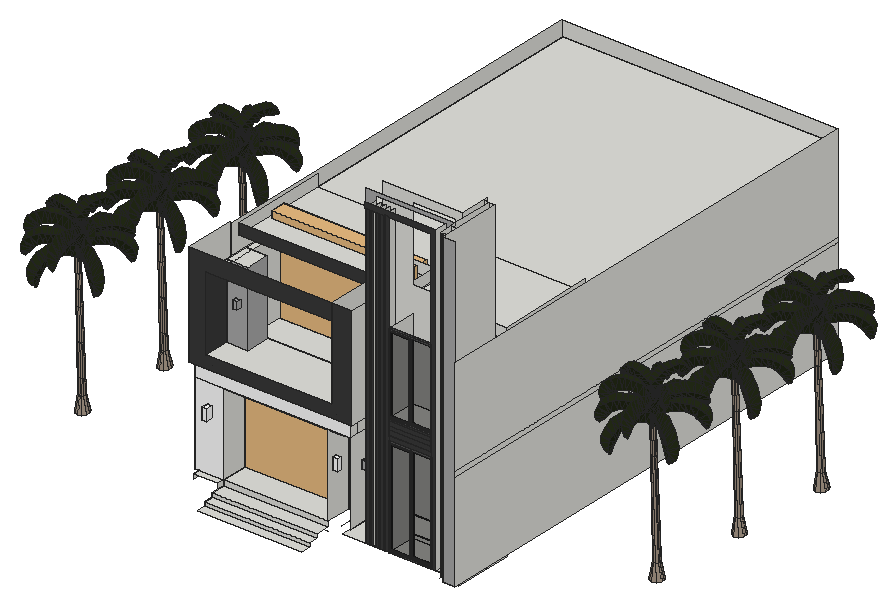
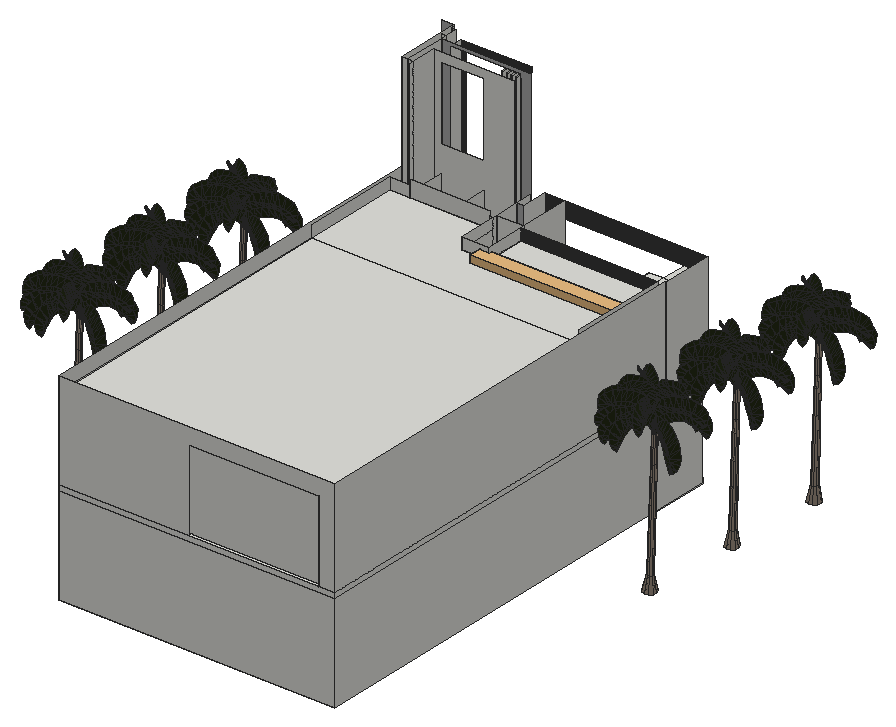
# SketchUp Ruby script. Lengths in inches.
U = 1.inch
M = Sketchup.active_model
def pt(a) = Geom::Point3d.new(a.map { |v| v * U })
def face(e, loops, mat)
  f = e.add_face(loops[0].map { |a| pt(a) })
  loops[1..].each { |l| e.add_face(l.map { |a| pt(a) }).erase! }
  f.material = f.back_material = mat if mat
  f
end
# faces: each face lists its corners as indices into pts; further lists are holes
def faces(e, pts, list, mat = nil) = list.each { |f| face(e, (f[0].is_a?(Array) ? f : [f]).map { |l| l.map { |i| pts[i] } }, mat) }
# xy, xz, yz: faces in a plane at the given z, y or x. An outline is a flat list of corners, or four numbers for a rectangle; further outlines are holes
def ring(l) = l.size == 4 ? [[l[0], l[1]], [l[2], l[1]], [l[2], l[3]], [l[0], l[3]]] : l.each_slice(2).to_a
def flat(e, list, mat, &to3) = list.each { |f| face(e, (f[0].is_a?(Array) ? f : [f]).map { |l| ring(l).map { |u, v| to3.(u, v) } }, mat) }
def xy(e, z, list, mat = nil) = flat(e, list, mat) { |x, y| [x, y, z] }
def xz(e, y, list, mat = nil) = flat(e, list, mat) { |x, z| [x, y, z] }
def yz(e, x, list, mat = nil) = flat(e, list, mat) { |y, z| [x, y, z] }
def lines(e, pts, list) = list.each { |a, b| e.add_line(pt(pts[a]), pt(pts[b])) }
# prism: a flat outline (further loops are holes) pulled along v
def prism(e, loops, v, mat = nil)
  f = face(e, loops, mat); d = Geom::Vector3d.new(v.map { |x| x * U })
  f.pushpull(f.normal.samedirection?(d) ? d.length : -d.length)
end
def box(e, o, s, mat = nil) = prism(e, [[o, [o[0] + s[0], o[1], o[2]], [o[0] + s[0], o[1] + s[1], o[2]], [o[0], o[1] + s[1], o[2]]]], [0, 0, s[2]], mat)
def at(x, y, z, deg = 0) = Geom::Transformation.translation(pt([x, y, z])) * Geom::Transformation.rotation(ORIGIN, Z_AXIS, deg.degrees)
def axes(o, x, y, z) = Geom::Transformation.new([*x, 0, *y, 0, *z, 0, *pt(o).to_a, 1])
def part(name) = M.definitions.add(name)
# library, detail: a bought-in or finely detailed component or shape, given as its bounding box
def library(name, o, s) = part(name).tap { |d| box(d.entities, o, s) }
def detail(e, o, s) = box(e.add_group.entities, o, s)
def put(e, d, t, mat = nil) = e.add_instance(d, t).tap { |i| i.material = mat if mat }
def group(e, t, mat = nil) = e.add_group.tap { |g| g.transformation = t; g.material = mat if mat }.entities
root = M.entities
M.materials.add("Glass_Tinted_Gray").color = [0, 0, 0]
M.materials["Glass_Tinted_Gray"].alpha = 0.125
M.materials.add("Manila2").color = [36, 43, 22]
M.materials.add("ManilaTruck").color = [158, 143, 128]
M.materials.add("[0135_DarkGray]").color = [81, 81, 81]
M.materials.add("[Color M00]").color = [255, 255, 255]
M.materials.add("[Color M03]").color = [170, 170, 170]
M.materials.add("[Color M06]").color = [86, 86, 86]
M.materials.add("[Color M07]").color = [58, 58, 58]
M.materials.add("[Mirror 02]").color = [229, 229, 229]
M.materials.add("[Terrazzo Light Blue]").color = [196, 214, 227]
c1 = part("P_trunck")
xz(c1.entities,2.71,[[7.39,73.15,8.49,73.15,9.26,91.63,8.16,91.63]],"ManilaTruck")
xz(c1.entities,6.09,[[3.91,10.2,7.39,73.15,8.49,73.15,5.33,10.2],[7.39,73.15,8.16,91.63,9.26,91.63,8.49,73.15]],"ManilaTruck")
p = [[3.19,0,0],[3.91,1.7,10.2],[2.75,2.54,10.2],[0.88,1.68,0],[6.05,0,0],[5.33,1.7,10.2],
  [8.36,1.68,0],[6.49,2.54,10.2],[2.31,3.9,10.2],[0,4.39,0],[9.24,4.39,0],[6.93,3.9,10.2],
  [2.75,5.25,10.2],[0.88,7.11,0],[8.36,7.11,0],[6.49,5.25,10.2],[3.91,6.09,10.2],[3.19,8.79,0],
  [6.05,8.79,0],[5.33,6.09,10.2],[7.39,2.71,73.15],[6.5,3.36,73.15],[8.49,2.71,73.15],[9.38,3.36,73.15],
  [6.16,4.4,73.15],[9.72,4.4,73.15],[6.5,5.45,73.15],[9.38,5.45,73.15],[7.39,6.09,73.15],[8.49,6.09,73.15],
  [8.16,2.71,91.63],[7.27,3.36,91.63],[10.15,3.36,91.63],[9.26,2.71,91.63],[6.93,4.4,91.63],[10.49,4.4,91.63],
  [7.27,5.45,91.63],[10.15,5.45,91.63],[8.16,6.09,91.63],[9.26,6.09,91.63]]
faces(c1.entities,p,[[0,1,2,3],[4,5,1,0],[6,7,5,4],[3,2,8,9],[6,10,11,7],[8,12,13,9],[11,10,14,15],[13,12,16,17],
  [18,19,15,14],[17,16,19,18],[1,20,21,2],[5,22,20,1],[7,23,22,5],[2,21,24,8],[7,11,25,23],[8,24,26,12],
  [11,15,27,25],[12,26,28,16],[19,29,27,15],[20,30,31,21],[23,32,33,22],[31,34,24,21],[23,25,35,32],[34,36,26,24],
  [25,27,37,35],[26,36,38,28],[29,39,37,27]],"ManilaTruck")
c2 = part("halfleave")
p = [[3.15,0,0],[0.57,2.5,1.86],[4.875,1.71,0],[46.16,1.62,0],[42.0625,6.98,0],[45.79,16.25,3.85],
  [48.16,12.12,1.98],[48.16,1.62,0],[6.6,3.42,0],[-0.25,5.68,3.48],[9.02,6.6,0],[-0.31,11.68,4.96],
  [2.05,16.625,5.9],[10.99,8.52,0],[36.71,10.67,0],[41.5,21.18,5.01],[8.2,21.17,6.52],[12.96,10.44,0],
  [15.16,24.88,6.8125],[17.61,12.89,0],[31.19,13.02,0],[36.16,23.66,5.26],[19.91,24.88,6.5625],[20.53,13.55,0],
  [25.77,13.9375,0],[30.57,24.88,6.0625],[25.21,24.88,6.26]]
faces(c2.entities,p,[[0,1,2],[3,4,5],[5,6,3],[7,3,6],[2,1,8],[9,8,1],[8,9,10],[11,10,9],
  [11,12,10],[13,10,12],[4,14,15],[15,5,4],[12,16,13],[17,13,16],[16,18,17],[19,17,18],
  [14,20,21],[21,15,14],[18,22,19],[23,19,22],[20,24,25],[25,21,20],[22,26,23],[24,23,26],
  [26,25,24]],"Manila2")
c3 = part("palmfronmanila")
put(c3.entities,c2,axes([0,0,4.06],[1,0,0],[0,1,0],[0,0,-1]))
put(c3.entities,c2,at(0,0,4.06))
c4 = part("manilafronnew")
put(c4.entities,c3,axes([0,16.76,11.56],[1,0,0],[0,0,1],[0,-1,0]))
c5 = part("Palm tree")
put(c5.entities,c1,axes([-10.55,-3.84,0],[1.24992,0,0],[0,1.28016,0],[0,0,1.424]))
g1 = group(c5.entities,at(-43.54,-39.32,114.59))
put(g1,c4,axes([4.6,65.71,26.23],[0.53953,-0.65683,-0.22776],[0.61942,0.58508,-0.22],[0.31564,-0.02543,0.82105]))
put(g1,c4,axes([82.14,44.18,-7.44],[-0.84198,0.16366,0.22983],[-0.16944,-0.87168,0],[0.22561,-0.04385,0.85774]))
put(g1,c4,axes([74.79,11.41,2.76],[-0.448,0.77596,0],[-0.77596,-0.448,0],[0,0,0.896]))
put(g1,c4,axes([70.64,6.04,20.22],[-0.30809,0.82895,-0.08038],[-0.79676,-0.31832,-0.22889],[-0.24248,-0.00729,0.85422]))
put(g1,c4,axes([56.04,79.09,38.5],[-0.31814,-0.55104,-0.36736],[0.63629,-0.36736,0],[-0.18368,-0.31814,0.63629]))
put(g1,c4,axes([8.39,50.1,50.01],[0.44591,-0.25744,-0.51489],[0.36408,0.63061,0],[0.44591,-0.25744,0.51489]))
put(g1,c4,axes([8.53,12.03,22.52],[0.79394,0.3635,-0.23397],[-0.37632,0.82195,0],[0.21274,0.0974,0.8732]))
put(g1,c4,axes([54.07,81.55,-7.16],[-0.44094,-0.76373,0.19874],[0.78289,-0.452,0],[0.09937,0.17211,0.88188]))
put(g1,c4,axes([11.98,71.79,5.35],[0.444,-0.76903,0],[0.76903,0.444,0],[0,0,0.888]))
put(g1,c4,axes([-0.47,46.08,5.17],[0.83758,-0.34011,0],[0.34011,0.83758,0],[0,0,0.904]))
put(g1,c4,axes([35.85,3.71,-10.8],[0.42686,0.73934,0.2973],[-0.78289,0.452,0],[-0.14865,-0.25747,0.85372]))
put(g1,c4,axes([0.28,29.91,5.17],[0.904,0,0],[0,0.904,0],[0,0,0.904]))
put(g1,c4,axes([82.45,61.59,11.57],[-0.88287,-0.17622,-0.08182],[0.17259,-0.88617,0.04625],[-0.08923,0.02954,0.8991]))
put(g1,c4,axes([59.47,9.58,46.3125],[-0.10851,0.51281,-0.52416],[-0.72522,-0.15346,0],[-0.10851,0.51281,0.52416]))
c6 = part("עצי+דקל")
put(c6.entities,c5,axes([111.95,22.91,0],[1.33,0,0],[0,1.33,0],[0,0,1.33]))
put(c6.entities,c5,axes([230.0625,22.91,0],[1.33,0,0],[0,1.33,0],[0,0,1.33]))
put(c6.entities,c5,axes([348.17,22.91,0],[1.33,0,0],[0,1.33,0],[0,0,1.33]))
c7 = part("PENTEK_RP Fineline 50S_Sliding_DoorCase_E1")
box(c7.entities,[0,0,0],[1.51,3.66,99.27],"[0135_DarkGray]")
c8 = part("PENTEK_RP Fineline 50S_SlidingDooe_Case_E2")
box(c8.entities,[0,0,0],[96.25,3.66,1.51],"[0135_DarkGray]")
c9 = part("pentek_RP Fineline 50S_SlidingDoor_Case")
put(c9.entities,c7,at(97.76,0,0))
put(c9.entities,c8,at(1.51,0,0))
put(c9.entities,c7,at(0,0,0))
put(c9.entities,c8,at(1.51,0,97.76))
c10 = part("PENTEK_RP Fineline 50S_SlidingDoor_GlazingBead_2")
box(c10.entities,[0,0,0],[0.56,0.59,94.39],"[0135_DarkGray]")
c11 = part("PENTEK_RP Fineline 50S_SlidingDoor_Glass")
box(c11.entities,[0,0,0],[46.58,0.16,94.39],"Glass_Tinted_Gray")
c12 = part("PENTEK_RP Fineline 50S_SlidingDoor_GlazingBead")
box(c12.entities,[0,0,0],[45.47,0.59,0.56],"[0135_DarkGray]")
c13 = part("PENTEK_RP Fineline 50S_SlidingDoor_Leaf_E1")
xy(c13.entities,0,[[0,0,0.93,1.97],[0.93,1.57,1.49,1.97]],"[0135_DarkGray]")
xy(c13.entities,96.25,[[0,0,0.93,0,0.93,1.57,1.49,1.57,1.49,1.97,0,1.97]],"[0135_DarkGray]")
xz(c13.entities,0,[[0,0,0.93,96.25]],"[0135_DarkGray]")
xz(c13.entities,1.57,[[0.93,0,1.49,95.32],[0.93,95.32,1.49,96.25]],"[0135_DarkGray]")
xz(c13.entities,1.97,[[0,0,1.49,96.25]],"[0135_DarkGray]")
yz(c13.entities,0,[[0,0,1.97,96.25]],"[0135_DarkGray]")
yz(c13.entities,0.93,[[0,0,1.57,0.93],[0,0.93,1.57,95.32],[0,95.32,1.57,96.25]],"[0135_DarkGray]")
yz(c13.entities,1.49,[[1.57,0,1.97,95.32],[1.57,95.32,1.97,96.25]],"[0135_DarkGray]")
c14 = part("PENTEK_RP Fineline 50S_SlidingDoor_Leaf_E2")
xy(c14.entities,0,[[0,0,0,1.57,0.56,1.57,0.56,1.97,46.02,1.97,46.02,1.57,46.58,1.57,46.58,0]],"[0135_DarkGray]")
xy(c14.entities,0.93,[[0,0,46.58,1.57]],"[0135_DarkGray]")
xy(c14.entities,1.49,[[0.56,1.57,46.02,1.97]],"[0135_DarkGray]")
xz(c14.entities,0,[[0,0,46.58,0.93]],"[0135_DarkGray]")
xz(c14.entities,1.57,[[0,0,0.56,0.93],[46.02,0,46.58,0.93],[0.56,0.93,46.02,1.49]],"[0135_DarkGray]")
xz(c14.entities,1.97,[[0.56,0,46.02,1.49]],"[0135_DarkGray]")
yz(c14.entities,0,[[0,0,1.57,0.93]],"[0135_DarkGray]")
yz(c14.entities,0.56,[[1.57,0,1.97,0.93],[1.57,0.93,1.97,1.49]],"[0135_DarkGray]")
yz(c14.entities,46.02,[[1.57,0,1.97,0.93],[1.57,0.93,1.97,1.49]],"[0135_DarkGray]")
yz(c14.entities,46.58,[[0,0,1.57,0.93]],"[0135_DarkGray]")
c15 = part("PENTEK_RP Fineline S_SlidingDoor_Leaf1")
put(c15.entities,c10,at(0.93,0,0.93))
put(c15.entities,c10,at(46.96,0,0.93))
put(c15.entities,c11,at(1.49,1.42,0.93))
put(c15.entities,c12,at(1.49,0,0.93))
put(c15.entities,c11,at(1.49,0.59,0.93),"[Terrazzo Light Blue]")
put(c15.entities,c13,at(0,0,0))
put(c15.entities,c13,axes([48.44,0,0],[-1,0,0],[0,1,0],[0,0,1]))
put(c15.entities,c14,axes([0.93,0,96.25],[1,0,0],[0,1,0],[0,0,-1]))
put(c15.entities,c14,at(0.93,0,0))
put(c15.entities,c12,at(1.49,0,94.77))
c16 = part("PENTEK_RP Fineline 50S_SlidingDoor_Leaf2")
put(c16.entities,c11,at(1.49,1.42,0.93))
put(c16.entities,c12,at(1.49,0,94.77))
put(c16.entities,c10,at(46.96,0,0.93))
put(c16.entities,c11,at(1.49,0.59,0.93),"[Mirror 02]")
put(c16.entities,c10,at(0.93,0,0.93))
put(c16.entities,c13,at(0,0,0))
put(c16.entities,c13,axes([48.44,0,0],[-1,0,0],[0,1,0],[0,0,1]))
put(c16.entities,c12,at(1.49,0,0.93))
put(c16.entities,c14,axes([0.93,0,96.25],[1,0,0],[0,1,0],[0,0,-1]))
put(c16.entities,c14,at(0.93,0,0))
c17 = part("PENTEK - Slimmest Steel Sliding Door / Window\#1")
put(c17.entities,c9,at(0,-1.88,-0.09))
put(c17.entities,c15,at(1.51,-2.27,1.42))
put(c17.entities,c16,at(49.32,-0.3,1.42))
c18 = library("Main+door",[0,-1.76,0],[126.77,13.57,114.16])
c19 = library("12",[112.18,111.43,0],[146.07,15.17,104.72])
xy(root,-16.8125,[[226.86,484.17,355.41,496.36]])
xy(root,-11.5,[[226.86,496.36,355.41,506.86]])
xy(root,-6.4375,[[226.86,506.86,355.41,524.55],[382.6,555.49,501.41,585.58],[501.41,555.49,525.63,585.58],[226.86,585.58,355.41,592.02]])
xy(root,0,[[515.78,500.24,515.78,512.52,525.63,512.52,525.63,1083.4,196.6875,1083.4,196.6875,524.55,191.6,524.55,191.6,1088.49,530.72,1088.49,530.72,500.24],[513.53,502.86,515.78,512.52],[508.41,505.61,513.53,512.52],[382.6,512.52,434.48,512.52,434.48,528.52,433.12,528.52,433.12,513.21,428.48,513.21,428.48,528.52,427.12,528.52,427.12,513.21,422.48,513.21,422.48,528.52,421.12,528.52,421.12,513.21,416.48,513.21,416.48,528.52,415.12,528.52,415.12,513.21,410.48,513.21,410.48,528.52,399.1,528.52,399.1,549.55,382.6,549.55],[434.48,512.52,439.12,512.52,439.12,549.55,399.1,549.55,399.1,528.52,410.48,528.52,410.48,513.21,415.12,513.21,415.12,528.52,416.48,528.52,416.48,513.21,421.12,513.21,421.12,528.52,422.48,528.52,422.48,513.21,427.12,513.21,427.12,528.52,428.48,528.52,428.48,513.21,433.12,513.21,433.12,528.52,434.48,528.52],
  [439.12,512.52,491.67,549.55],[491.67,512.52,491.67,549.55,501.41,549.55,501.41,528.52,497.28,528.52,497.28,512.52],[497.28,512.52,501.41,528.52],[501.41,512.52,508.41,528.52],[508.41,512.52,513.53,521.24],
  [513.53,512.52,513.53,521.24,508.41,521.24,508.41,555.49,515.78,555.49,515.78,512.52],[515.78,512.52,525.63,555.49],[196.6875,516.27,226.86,524.55],[196.6875,524.55,226.86,585.58],[226.86,524.55,355.41,585.58],
  [501.41,528.52,508.41,555.49],[382.6,549.55,501.41,555.49],[355.41,555.49,371.29,585.58],[371.29,555.49,382.6,585.58],[382.6,555.49,501.41,585.58],
  [501.41,555.49,508.41,580.49],[515.78,555.49,525.63,555.49,525.63,585.58,501.41,585.58,501.41,580.49,515.78,580.49],[508.41,555.49,515.78,580.49],[196.6875,585.58,226.86,585.58,226.86,592.02,355.41,592.02,355.41,585.58,525.63,585.58,525.63,1083.4,196.6875,1083.4],[226.86,585.58,355.41,592.02]])
xy(root,61.39,[[364.57,519.74,370.5,524.55]],"[Color M00]")
xy(root,62.82,[[207.32,515.86,212.94,524.55]],"[Color M00]")
xy(root,63.5625,[[388.03,535.86,394.15,549.55]],"[Color M03]")
xy(root,73.47,[[388.03,535.86,394.15,549.55]],"[Color M03]")
xy(root,75.82,[[364.57,519.74,370.5,524.55]],"[Color M00]")
xy(root,76.75,[[207.32,515.86,212.94,524.55]],"[Color M00]")
xy(root,100.625,[[226.86,524.55,355.41,585.58],[355.41,524.55,371.29,536.49],[371.29,524.55,382.6,536.49],[355.41,536.49,371.29,555.49],[371.29,536.49,382.6,555.49]])
xy(root,120,[[189.35,517.74,189.35,536.49,191.6,536.49,191.6,524.55,380.7,524.55,380.7,517.74],[380.7,517.74,380.7,524.55,382.6,524.55,382.6,536.49,390.22,536.49,390.22,517.74],[191.6,524.55,380.7,536.49],[380.7,524.55,382.6,536.49],[189.35,536.49,191.6,580.49],
  [191.6,536.49,380.7,580.49],[380.7,536.49,382.6,580.49],[382.6,536.49,390.22,549.55],[382.6,549.55,399.1,580.49],[382.6,580.49,399.1,585.58],
  [196.6875,585.58,525.63,1083.4]])
xy(root,123.125,[[439.12,512.52,491.67,549.55]])
xy(root,126,[[210.67,580.49,365.35,585.58],[365.35,580.49,371.29,585.58],[371.29,580.49,399.1,585.58],[196.6875,585.58,210.67,706.36],[210.67,585.58,365.35,585.58,365.35,634.36,371.29,634.36,371.29,1083.4,210.67,1083.4],
  [365.35,585.58,371.29,634.36],[371.29,585.58,399.1,634.36],[399.1,585.58,525.63,585.58,525.63,706.36,371.29,706.36,371.29,634.36,399.1,634.36],[196.6875,706.36,210.67,1083.4],[371.29,706.36,525.63,1083.4],
  [210.67,1083.4,371.29,1088.49]])
xy(root,128.59,[[439.12,512.52,491.67,513.21]])
xy(root,134.9375,[[210.67,517.74,365.35,517.74,365.35,580.49,210.67,580.49,210.67,578.99,236.67,578.99,236.67,549.11,210.67,549.11],[210.67,549.11,236.67,578.99]])
xy(root,147.83,[[439.12,513.21,491.67,577.96]])
xy(root,178.34,[[221.88,544.3,227.76,549.11]],"[Color M03]")
xy(root,187.84,[[221.88,544.3,227.76,549.11]],"[Color M03]")
xy(root,226.5625,[[210.67,517.74,218.17,549.11],[210.67,549.11,218.17,578.99],[218.17,549.11,236.67,578.99],[210.67,578.99,218.17,1088.49]])
xy(root,232.125,[[196.6875,585.58,196.6875,706.36,525.63,706.36,525.63,585.58,399.1,585.58,399.1,634.36,365.35,634.36,365.35,585.58],[196.6875,706.36,525.63,1083.4]])
xz(root,496.36,[[226.86,-16.8125,355.41,-11.5]])
xz(root,500.24,[[515.78,0,530.72,379.5625]],"[Color M03]")
xz(root,502.86,[[513.53,0,515.78,379.5625]],"[Color M03]")
xz(root,505.61,[[508.41,0,513.53,379.5625]],"[Color M03]")
xz(root,506.86,[[226.86,-11.5,355.41,-6.4375]])
xz(root,512.52,[[491.67,0,497.28,0,497.28,375.375,410.48,375.375,410.48,369.375,491.67,369.375],[434.48,0,439.12,369.375],[439.12,123.125,491.67,128.59]],"[Color M07]")
xz(root,513.21,[[410.48,0,415.12,369.375],[416.48,0,421.12,369.375],[422.48,0,427.12,369.375],[428.48,0,433.12,369.375],[439.12,128.59,491.67,134.05],
  [439.12,134.05,491.67,139.45],[439.12,139.45,491.67,144.31],[439.12,144.31,491.67,147.83]],"[Color M07]")
xz(root,515.86,[[207.32,62.82,212.94,76.75]],"[Color M00]")
xz(root,517.74,[[189.35,120,390.22,120,390.22,246,365.35,246,365.35,134.9375,210.67,134.9375,210.67,226.5625,365.35,226.5625,365.35,246,189.35,246]],"[Color M07]")
xz(root,519.74,[[364.57,61.39,370.5,75.82]],"[Color M00]")
xz(root,521.24,[[508.41,0,513.53,379.5625]])
xz(root,524.55,[[226.86,-6.4375,355.41,0]])
xz(root,524.55,[[[191.6,0,226.86,100.625],[207.32,62.82,212.94,76.75]],[191.6,100.625,382.6,120]],"[Color M00]")
xz(root,528.52,[[415.12,0,416.48,369.375],[421.12,0,422.48,369.375],[427.12,0,428.48,369.375],[433.12,0,434.48,369.375]])
xz(root,528.52,[[399.1,0,410.48,0,410.48,375.375,497.28,375.375,497.28,0,508.41,0,508.41,379.5625,398.66,379.5625,398.66,252,398.6,252,398.6,246,399.1,246]],"[Color M03]")
xz(root,535.86,[[388.03,63.5625,394.15,73.47]],"[Color M03]")
xz(root,544.3,[[221.88,178.34,227.76,187.84]],"[Color M03]")
xz(root,549.11,[[[210.67,134.9375,236.67,226.5625],[221.88,178.34,227.76,187.84]]],"[Color M03]")
xz(root,549.55,[[[399.1,0,399.1,246,402.91,246,402.91,379.5625,501.41,379.5625,501.41,0,491.67,0,491.67,123.125,439.12,123.125,439.12,0],[439.12,278.25,491.67,369.375]]])
xz(root,549.55,[[[382.6,0,399.1,120],[388.03,63.5625,394.15,73.47]],[390.22,120,399.1,246]],"[Color M03]")
xz(root,555.49,[[382.6,-6.4375,501.41,0],[501.41,-6.4375,525.63,0],[355.41,0,382.6,100.625]])
xz(root,577.96,[[439.12,147.83,491.67,246.25]])
xz(root,578.99,[[210.67,134.9375,236.67,226.5625]])
xz(root,580.49,[[501.41,0,508.41,379.5625],[508.41,0,515.78,379.5625],[189.35,120,191.6,126],[191.6,120,399.1,126],[189.35,126,191.6,246],
  [210.67,126,365.35,134.9375],[365.35,126,399.1,246]])
xz(root,585.58,[[226.86,-16.8125,355.41,-11.5],[226.86,-11.5,355.41,-6.4375],[196.6875,-6.4375,226.86,0],[226.86,-6.4375,355.41,0],[382.6,-6.4375,501.41,0],
  [501.41,-6.4375,525.63,0],[196.6875,0,196.6875,120,382.6,120,382.6,0,355.41,0,355.41,100.625,226.86,100.625,226.86,0],[382.6,0,501.41,120],[501.41,0,525.63,120],[399.1,120,501.41,126],
  [399.1,126,501.41,232.125],[399.1,232.125,402.91,246],[402.91,232.125,501.41,252],[501.41,232.125,525.63,246]])
xz(root,585.58,[[196.6875,232.125,365.35,246]],"[Color M07]")
xz(root,592.02,[[226.86,-6.4375,355.41,0]])
xz(root,634.36,[[365.35,126,399.1,232.125],[365.35,232.125,399.1,246]])
xz(root,1083.4,[[196.6875,0,525.63,120],[196.6875,126,525.63,232.125]])
xz(root,1088.49,[[191.6,0,530.72,120],[191.6,120,530.72,126],[191.6,126,191.6,246,530.72,246,530.72,126,371.29,126,371.29,226.5625,210.67,226.5625,210.67,126]])
yz(root,189.35,[[517.74,120,580.49,246]])
yz(root,191.6,[[524.55,0,524.55,100.625,536.49,100.625,536.49,120,1088.49,120,1088.49,0],[524.55,100.625,536.49,120],[580.49,120,1088.49,126],[580.49,126,1088.49,246]])
yz(root,196.6875,[[516.27,-6.4375,585.58,0],[585.58,0,1083.4,120],[706.36,126,1083.4,232.125],[585.58,232.125,706.36,246]])
yz(root,207.32,[[515.86,62.82,524.55,76.75]],"[Color M00]")
yz(root,210.67,[[580.49,126,1088.49,126,1088.49,226.5625,578.99,226.5625,578.99,134.9375,580.49,134.9375],[549.11,134.9375,578.99,226.5625]])
yz(root,210.67,[[517.74,134.9375,549.11,226.5625]],"[Color M07]")
yz(root,212.94,[[515.86,62.82,524.55,76.75]],"[Color M00]")
yz(root,221.88,[[544.3,178.34,549.11,187.84]],"[Color M03]")
yz(root,226.86,[[496.36,-16.8125,516.27,-11.5],[516.27,-16.8125,524.55,-11.5],[524.55,-16.8125,555.49,-11.5],[555.49,-16.8125,585.58,-11.5],[506.86,-11.5,516.27,-6.4375],
  [516.27,-11.5,524.55,-6.4375],[524.55,-11.5,555.49,-6.4375],[555.49,-11.5,585.58,-6.4375],[516.27,-6.4375,524.55,0],[524.55,-6.4375,585.58,0],
  [585.58,-6.4375,592.02,0],[524.55,0,585.58,100.625]])
yz(root,227.76,[[544.3,178.34,549.11,187.84]],"[Color M03]")
yz(root,236.67,[[549.11,134.9375,578.99,226.5625]],"[Color M03]")
yz(root,355.41,[[585.58,-6.4375,592.02,0],[524.55,0,555.49,100.625],[555.49,0,585.58,100.625]])
yz(root,364.57,[[519.74,61.39,524.55,75.82]],"[Color M00]")
yz(root,365.35,[[580.49,126,580.49,246,585.58,246,585.58,232.125,634.36,232.125,634.36,126],[517.74,134.9375,580.49,246],[585.58,232.125,634.36,246]])
yz(root,370.5,[[519.74,61.39,524.55,75.82]],"[Color M00]")
yz(root,382.6,[[524.55,-6.4375,555.49,0],[555.49,-6.4375,585.58,0],[524.55,0,549.55,100.625],[549.55,0,555.49,100.625],[555.49,0,585.58,0,585.58,120,549.55,120,549.55,100.625,555.49,100.625],
  [524.55,100.625,536.49,120],[536.49,100.625,549.55,120]])
yz(root,388.03,[[535.86,63.5625,549.55,73.47]],"[Color M03]")
yz(root,390.22,[[517.74,120,549.55,246]])
yz(root,394.15,[[535.86,63.5625,549.55,73.47]],"[Color M03]")
yz(root,399.1,[[528.52,0,549.55,246],[549.55,120,580.49,126],[580.49,120,585.58,126],[549.55,126,580.49,246],[580.49,126,585.58,246],
  [585.58,126,634.36,232.125],[585.58,232.125,634.36,246]])
yz(root,410.48,[[513.21,0,528.52,369.375]])
yz(root,415.12,[[513.21,0,528.52,369.375]])
yz(root,416.48,[[513.21,0,528.52,369.375]])
yz(root,421.12,[[513.21,0,528.52,369.375]])
yz(root,422.48,[[513.21,0,528.52,369.375]])
yz(root,427.12,[[513.21,0,528.52,369.375]])
yz(root,428.48,[[513.21,0,528.52,369.375]])
yz(root,433.12,[[513.21,0,528.52,369.375]])
yz(root,434.48,[[512.52,0,528.52,369.375]])
yz(root,439.12,[[512.52,0,549.55,123.125],[512.52,128.59,513.21,134.05],[512.52,134.05,513.21,139.45],[512.52,139.45,513.21,144.31],[512.52,144.31,513.21,147.83],
  [512.52,147.83,577.96,246.25]])
yz(root,491.67,[[512.52,0,549.55,123.125],[512.52,128.59,513.21,134.05],[512.52,134.05,513.21,139.45],[512.52,139.45,513.21,144.31],[512.52,144.31,513.21,147.83],
  [512.52,147.83,577.96,246.25]])
yz(root,497.28,[[512.52,0,528.52,375.375]])
yz(root,501.41,[[555.49,-6.4375,585.58,0],[549.55,0,580.49,379.5625],[580.49,0,585.58,379.5625]])
yz(root,508.41,[[505.61,0,521.24,379.5625],[521.24,0,528.52,379.5625],[528.52,0,580.49,379.5625]])
yz(root,513.53,[[502.86,0,505.61,379.5625]])
yz(root,515.78,[[500.24,0,502.86,379.5625],[502.86,0,580.49,379.5625]])
yz(root,525.63,[[512.52,-6.4375,555.49,0],[555.49,-6.4375,585.58,0],[585.58,0,1083.4,120],[706.36,126,1083.4,232.125],[585.58,232.125,706.36,246]])
yz(root,530.72,[[500.24,0,1088.49,120],[500.24,120,1088.49,126],[500.24,126,1088.49,246]])
p = [[218.17,549.11,126],[218.17,517.74,126],[371.29,549.11,126],[371.29,517.74,126],[365.35,549.11,126],[501.41,555.49,-6.4375],
  [501.41,512.52,-6.4375],[226.86,524.55,-11.5],[355.41,524.55,-11.5],[371.29,555.49,0],[371.29,524.55,0]]
lines(root,p,[[0,1],[2,3],[2,4],[5,6],[7,8],[9,10]])
put(root,c6,at(658.14,986.55,-7.35,-93.2))
put(root,c17,axes([439.92,514.4,0.11],[0.52935,0,0],[0,1,0],[0,0,1.24028]))
put(root,c18,axes([228.64,557.02,1.31],[1,0,0],[0,0.87,0],[0,0,0.87]),"[Color M07]")
put(root,c6,at(55.16,857.67,21.2,-93.2))
put(root,c19,axes([64.66,496.4,126],[1.2096,0,0],[0,1.2096,0],[0,0,1.09337]),"[Color M06]")
put(root,c17,axes([439.12,514.4,147.7],[0.52935,0,0],[0,1,0],[0,0,0.9936]))
